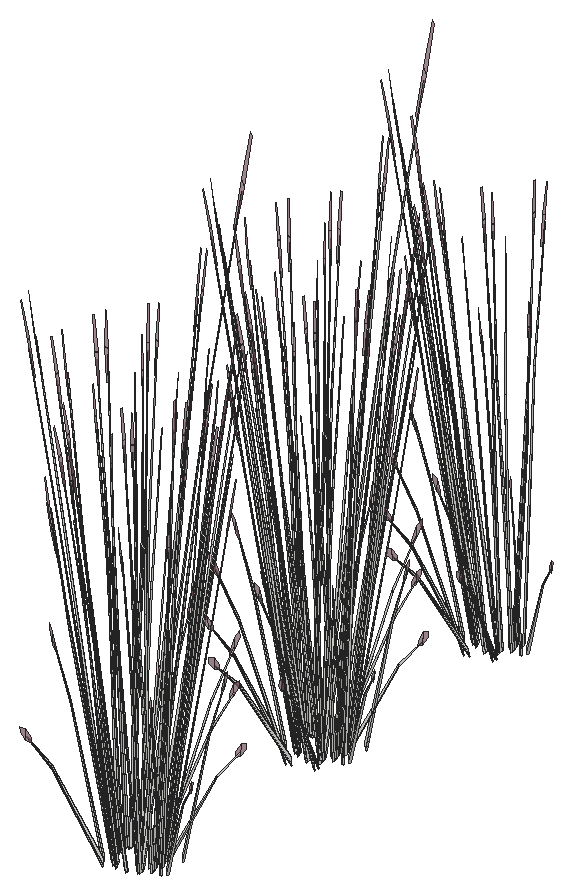
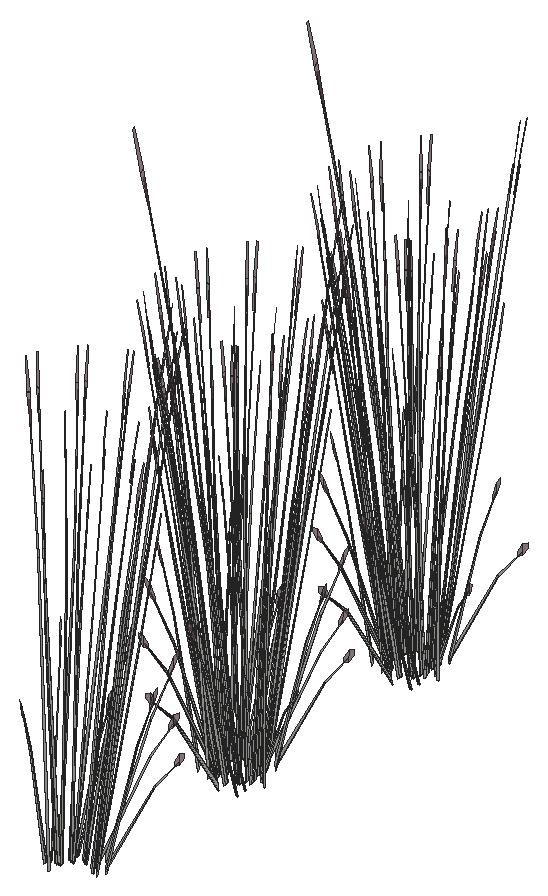
# SketchUp Ruby script. Lengths in inches.
U = 1.inch
M = Sketchup.active_model
def pt(a) = Geom::Point3d.new(a.map { |v| v * U })
def face(e, loops, mat)
  f = e.add_face(loops[0].map { |a| pt(a) })
  loops[1..].each { |l| e.add_face(l.map { |a| pt(a) }).erase! }
  f.material = f.back_material = mat if mat
  f
end
# faces: each face lists its corners as indices into pts; further lists are holes
def faces(e, pts, list, mat = nil) = list.each { |f| face(e, (f[0].is_a?(Array) ? f : [f]).map { |l| l.map { |i| pts[i] } }, mat) }
# xy, xz, yz: faces in a plane at the given z, y or x. An outline is a flat list of corners, or four numbers for a rectangle; further outlines are holes
def ring(l) = l.size == 4 ? [[l[0], l[1]], [l[2], l[1]], [l[2], l[3]], [l[0], l[3]]] : l.each_slice(2).to_a
def flat(e, list, mat, &to3) = list.each { |f| face(e, (f[0].is_a?(Array) ? f : [f]).map { |l| ring(l).map { |u, v| to3.(u, v) } }, mat) }
def xy(e, z, list, mat = nil) = flat(e, list, mat) { |x, y| [x, y, z] }
def xz(e, y, list, mat = nil) = flat(e, list, mat) { |x, z| [x, y, z] }
def yz(e, x, list, mat = nil) = flat(e, list, mat) { |y, z| [x, y, z] }
def lines(e, pts, list) = list.each { |a, b| e.add_line(pt(pts[a]), pt(pts[b])) }
# prism: a flat outline (further loops are holes) pulled along v
def prism(e, loops, v, mat = nil)
  f = face(e, loops, mat); d = Geom::Vector3d.new(v.map { |x| x * U })
  f.pushpull(f.normal.samedirection?(d) ? d.length : -d.length)
end
def box(e, o, s, mat = nil) = prism(e, [[o, [o[0] + s[0], o[1], o[2]], [o[0] + s[0], o[1] + s[1], o[2]], [o[0], o[1] + s[1], o[2]]]], [0, 0, s[2]], mat)
def at(x, y, z, deg = 0) = Geom::Transformation.translation(pt([x, y, z])) * Geom::Transformation.rotation(ORIGIN, Z_AXIS, deg.degrees)
def axes(o, x, y, z) = Geom::Transformation.new([*x, 0, *y, 0, *z, 0, *pt(o).to_a, 1])
def part(name) = M.definitions.add(name)
# library, detail: a bought-in or finely detailed component or shape, given as its bounding box
def library(name, o, s) = part(name).tap { |d| box(d.entities, o, s) }
def detail(e, o, s) = box(e.add_group.entities, o, s)
def put(e, d, t, mat = nil) = e.add_instance(d, t).tap { |i| i.material = mat if mat }
def group(e, t, mat = nil) = e.add_group.tap { |g| g.transformation = t; g.material = mat if mat }.entities
root = M.entities
M.materials.add("LightPink_Translucent").color = [144, 107, 117]
M.materials["LightPink_Translucent"].alpha = 0.75
c1 = part("blade")
p = [[2.15,0.21,22],[0,0.17,0],[0.09,0.45,0],[2.18,0.31,22],[2.29,0.31,22],[0.38,0.45,0],
  [2.48,0.24,33],[2.49,0.24,33],[2.48,0.22,33]]
faces(c1.entities,p,[[0,1,2,3],[4,5,2,3],[6,3,4,7],[8,0,3,6]])
c2 = part("seeds")
p = [[0.3,-0.1,1.38],[-0.01,-0.03,1.59],[-0.01,-0.03,0.03],[0.14,-0.07,-0.07],[0.29,-0.03,3],[0.15,0.01,3.11]]
faces(c2.entities,p,[[0,1,2,3],[1,0,4,5]],"LightPink_Translucent")
c3 = part("blade with seeds")
put(c3.entities,c1,at(0,0,0))
put(c3.entities,c2,axes([2.4,0.25,30.99],[1.5799,-0.05474,1.17369],[-0.12525,1.92788,0.29478],[-0.07173,-0.02425,1.56792]))
put(root,c3,axes([402.43,636.52,4.73],[0.26007,-0.1585,0.0643],[0.12729,0.28902,0.50621],[-0.02512,-0.1274,0.77189]))
put(root,c3,axes([401.54,636.56,4.73],[0.16041,-0.29625,0.0643],[0.22843,0.17248,0.50621],[-0.07385,-0.09498,0.77189]))
put(root,c3,axes([402.33,636.84,5.05],[-0.1064,0.35863,0.35414],[-0.31043,-0.1046,-0.4572],[-0.02846,-0.14439,0.87481]))
put(root,c3,axes([403.125,636.99,4.73],[0.25132,0.3182,0.48003],[-0.2669,0.27442,0.3958],[0.04636,-0.14929,0.9933]))
put(root,c3,axes([401.61,636.53,5.43],[-0.23555,0.44708,-0.13619],[-0.34112,-0.25757,-0.75594],[-0.11858,-0.12631,1.14864]))
put(root,c3,axes([403.22,637.02,4.73],[0.29004,0.02173,0.0643],[-0.00795,0.32812,0.50621],[0.03035,-0.12569,0.77189]))
put(root,c3,axes([403,637.24,5.05],[-0.23881,0.24554,0.35414],[-0.22606,-0.28036,-0.4572],[0.0344,-0.14245,0.87481]))
put(root,c3,axes([400.71,636.4,4.72],[-0.07594,-0.00329,1.74944],[-0.24177,0.32918,-0.27667],[-0.129,-0.06726,0.14031]))
put(root,c3,axes([403.58,638.04,5.03],[-0.32648,-0.25715,-0.1216],[0.18809,-0.3724,-0.67495],[0.09224,-0.12945,1.02557]))
put(root,c3,axes([401.59,636.9,5.05],[0.05451,0.37564,0.35414],[-0.31161,0.09919,-0.4572],[-0.0837,-0.10765,0.87481]))
put(root,c3,axes([400.65,637.15,5.09],[0.29147,-0.34417,0.53763],[0.25138,0.3655,0.4433],[-0.13675,-0.06349,1.11249]))
put(root,c3,axes([404.38,637.93,4.71],[-0.0461,-0.00354,1.77383],[-0.19143,-0.37951,-0.16761],[0.07688,-0.12478,0.31391]))
put(root,c3,axes([400.78,637.14,4.73],[0.01777,-0.35463,0.0643],[0.26836,0.00972,0.50621],[-0.1028,-0.03711,0.77189]))
put(root,c3,axes([403.42,638,5.05],[-0.30722,0.06665,0.35414],[-0.08112,-0.381,-0.4572],[0.08804,-0.10234,0.87481]))
put(root,c3,axes([403.7,637.94,4.73],[0.2423,0.19613,0.0643],[-0.14107,0.2793,0.50621],[0.07768,-0.0903,0.77189]))
put(root,c3,axes([403.63,637.86,4.73],[0.08753,0.42921,0.48003],[-0.34336,0.07449,0.3958],[0.1012,-0.10094,0.9933]))
put(root,c3,axes([404.55,638.38,4.72],[0.04898,-0.07104,1.74944],[-0.06269,-0.43574,-0.27667],[0.12289,-0.08262,0.14031]))
put(root,c3,axes([400.42,636.68,4.71],[0.02617,0.04654,1.77383],[-0.12614,0.41836,-0.16761],[-0.12775,0.00303,0.31391]))
put(root,c3,axes([400.97,637.41,5.05],[0.20082,0.29199,0.35414],[-0.2293,0.2764,-0.4572],[-0.1165,-0.04206,0.87481]))
put(root,c3,axes([400.91,637.22,5.03],[-0.0189,0.47427,-0.1216],[-0.35781,-0.01296,-0.67495],[-0.13781,-0.03295,1.02557]))
put(root,c3,axes([403.59,639.04,5.03],[-0.17758,-0.42229,-0.1216],[0.31518,-0.20752,-0.67495],[0.13282,-0.05572,1.02557]))
put(root,c3,axes([403.47,638.91,5.05],[-0.29332,-0.1301,0.35414],[0.08555,-0.37955,-0.4572],[0.11809,-0.0348,0.87481]))
put(root,c3,axes([400.4,638.22,4.73],[0.09971,-0.42522,0.48003],[0.32782,0.1454,0.3958],[-0.12892,0.02555,0.9933]))
put(root,c3,axes([400.37,638.11,4.73],[-0.12963,-0.31798,0.0643],[0.23638,-0.15564,0.50621],[-0.1042,0.03071,0.77189]))
put(root,c3,axes([403.73,639.03,4.73],[0.12963,0.31798,0.0643],[-0.23638,0.15564,0.50621],[0.1042,-0.03071,0.77189]))
put(root,c3,axes([403.71,638.92,4.73],[-0.09971,0.42522,0.48003],[-0.32782,-0.1454,0.3958],[0.12892,-0.02555,0.9933]))
put(root,c3,axes([400.64,638.23,5.05],[0.29332,0.1301,0.35414],[-0.08555,0.37955,-0.4572],[-0.11809,0.0348,0.87481]))
put(root,c3,axes([404.3,640.3,4.71],[-0.03191,-0.04083,1.77383],[0.06981,-0.43764,-0.16761],[0.12571,-0.02796,0.31391]))
put(root,c3,axes([400.14,638.52,4.72],[-0.05763,0.06055,1.74944],[0.0049,0.44239,-0.27667],[-0.13211,0.05753,0.14031]))
put(root,c3,axes([400.51,638.1,5.03],[0.17758,0.42229,-0.1216],[-0.31518,0.20752,-0.67495],[-0.13282,0.05572,1.02557]))
put(root,c3,axes([403.19,639.92,5.03],[0.0189,-0.47427,-0.1216],[0.35781,0.01296,-0.67495],[0.13781,0.03295,1.02557]))
put(root,c3,axes([403.14,639.73,5.05],[-0.20082,-0.29199,0.35414],[0.2293,-0.2764,-0.4572],[0.1165,0.04206,0.87481]))
put(root,c3,axes([403.5,639.63,4.72],[0.07571,-0.00789,1.74944],[0.20767,-0.36231,-0.27667],[0.13467,0.04783,0.14031]))
put(root,c3,axes([400.47,639.28,4.73],[-0.08753,-0.42921,0.48003],[0.34336,-0.07449,0.3958],[-0.1012,0.10094,0.9933]))
put(root,c3,axes([400.41,639.2,4.73],[-0.2423,-0.19613,0.0643],[0.14107,-0.2793,0.50621],[-0.07768,0.0903,0.77189]))
put(root,c3,axes([400.6875,639.14,5.05],[0.30722,-0.06665,0.35414],[0.08112,0.381,-0.4572],[-0.08804,0.10234,0.87481]))
put(root,c3,axes([399.5,638.97,4.71],[0.04504,0.01251,1.77383],[0.13934,0.41205,-0.16761],[-0.0922,0.10815,0.31391]))
put(root,c3,axes([403.32,640,4.73],[-0.01777,0.35463,0.0643],[-0.26836,-0.00972,0.50621],[0.1028,0.03711,0.77189]))
put(root,c3,axes([403.34,639.89,4.73],[-0.26024,0.30729,0.48003],[-0.22444,-0.32634,0.3958],[0.1221,0.05668,0.9933]))
put(root,c3,axes([399.99,640.22,5.65],[0.31145,0.12449,-0.06488],[-0.0958,0.38314,-0.29416],[-0.05094,0.05817,0.97024]))
put(root,c3,axes([402.52,640.24,5.05],[-0.05451,-0.37564,0.35414],[0.31161,-0.09919,-0.4572],[0.0837,0.10765,0.87481]))
put(root,c3,axes([402.72,638.08,4.47],[-0.30498,-0.24231,1.38283],[0.32203,-0.37727,0.59665],[0.0984,0.22736,1.33663]))
put(root,c3,axes([400.53,639.1,5.03],[0.32648,0.25715,-0.1216],[-0.18809,0.3724,-0.67495],[-0.09224,0.12945,1.02557]))
put(root,c3,axes([402.49,640.44,5.03],[0.21031,-0.39918,-0.1216],[0.30457,0.22997,-0.67495],[0.10587,0.11278,1.02557]))
put(root,c3,axes([401.1,639.9,5.05],[0.23881,-0.24554,0.35414],[0.22606,0.28036,-0.4572],[-0.0344,0.14245,0.87481]))
put(root,c3,axes([402.21,640.77,4.71],[0.00104,-0.05646,1.77383],[0.30246,-0.2491,-0.16761],[0.10506,0.08891,0.31391]))
put(root,c3,axes([400.88,640.12,4.73],[-0.29004,-0.02173,0.0643],[0.00795,-0.32812,0.50621],[-0.03035,0.12569,0.77189]))
put(root,c3,axes([400.98,640.15,4.73],[-0.25132,-0.3182,0.48003],[0.2669,-0.27442,0.3958],[-0.04636,0.14929,0.9933]))
put(root,c3,axes([401.77,640.3,5.05],[0.1064,-0.35863,0.35414],[0.31043,0.1046,-0.4572],[0.02846,0.14439,0.87481]))
put(root,c3,axes([402.56,640.58,4.73],[-0.16041,0.29625,0.0643],[-0.22843,-0.17248,0.50621],[0.07385,0.09498,0.77189]))
put(root,c3,axes([402.1875,641.58,5.65],[0.2439,-0.26754,-0.06488],[0.22348,0.29302,-0.29416],[0.01573,0.08303,0.97024]))
put(root,c3,axes([402.63,640.5,4.73],[-0.35104,0.10702,0.48003],[-0.06092,-0.41983,0.3958],[0.08256,0.12373,0.9933]))
put(root,c3,axes([401.67,640.625,4.73],[-0.26007,0.1585,0.0643],[-0.12729,-0.28902,0.50621],[0.02512,0.1274,0.77189]))
put(root,c3,axes([400.15,640.17,4.72],[-0.00877,0.09229,1.74944],[0.24897,0.32105,-0.27667],[-0.06518,0.15182,0.14031]))
put(root,c3,axes([400.95,639.96,5.4],[0.3879,0.02311,-0.13498],[-0.0106,0.43749,-0.74919],[-0.02694,0.1685,1.13838]))
put(root,c3,axes([401.67,640.45,5.03],[0.34538,-0.21713,-0.1216],[0.16972,0.38536,-0.67495],[0.04557,0.16239,1.02557]))
put(root,c3,axes([401.77,640.6,5.0625],[-0.34777,-0.12192,0.53283],[0.11892,-0.40083,0.43934],[0.0209,0.15763,1.10256]))
put(root,c3,axes([400.125,641.12,4.71],[0.04004,-0.02816,1.77383],[0.33095,0.18728,-0.16761],[-0.00778,0.15594,0.31391]))
put(root,c3,axes([401.58,641.3125,4.72],[0.04474,0.0751,1.74944],[0.36104,0.0295,-0.27667],[0.03631,0.16562,0.14031]))
put(root,c3,axes([401.89,654.35,4.72],[-0.05398,-0.06539,1.74944],[-0.36026,0.04145,-0.27667],[-0.0575,-0.15639,0.14031]))
put(root,c3,axes([403.51,655.16,4.72],[-0.00341,-0.09282,1.74944],[-0.28775,-0.26825,-0.27667],[0.04449,-0.16261,0.14031]))
put(root,c3,axes([403.43,654.82,4.71],[-0.03584,0.03562,1.77383],[-0.35118,-0.12018,-0.16761],[-0.01271,-0.15545,0.31391]))
put(root,c3,axes([401.52,654.14,4.71],[-0.00658,0.0559,1.77383],[-0.32474,0.20287,-0.16761],[-0.09556,-0.1037,0.31391]))
put(root,c3,axes([401.45,655.13,5.09],[0.39316,-0.11987,0.53763],[0.06823,0.47021,0.4433],[-0.09247,-0.13858,1.11249]))
put(root,c3,axes([402.34,655.22,4.73],[0.34777,0.12192,0.48003],[-0.11892,0.40083,0.3958],[-0.0209,-0.15763,0.9933]))
put(root,c3,axes([402.4375,655.36,5.03],[-0.34538,0.21713,-0.1216],[-0.16972,-0.38536,-0.67495],[-0.04557,-0.16239,1.02557]))
put(root,c3,axes([403.15,655.85,5.03],[-0.3879,-0.02311,-0.1216],[0.0106,-0.43749,-0.67495],[0.02694,-0.1685,1.02557]))
put(root,c3,axes([402.43,655.19,4.73],[0.26007,-0.1585,0.0643],[0.12729,0.28902,0.50621],[-0.02512,-0.1274,0.77189]))
put(root,c3,axes([401.54,655.23,4.73],[0.16041,-0.29625,0.0643],[0.22843,0.17248,0.50621],[-0.07385,-0.09498,0.77189]))
put(root,c3,axes([402.33,655.51,5.05],[-0.1064,0.35863,0.35414],[-0.31043,-0.1046,-0.4572],[-0.02846,-0.14439,0.87481]))
put(root,c3,axes([403.125,655.67,4.73],[0.25132,0.3182,0.48003],[-0.2669,0.27442,0.3958],[0.04636,-0.14929,0.9933]))
put(root,c3,axes([401.61,655.2,5.43],[-0.23555,0.44708,-0.13619],[-0.34112,-0.25757,-0.75594],[-0.11858,-0.12631,1.14864]))
put(root,c3,axes([403.22,655.7,4.73],[0.29004,0.02173,0.0643],[-0.00795,0.32812,0.50621],[0.03035,-0.12569,0.77189]))
put(root,c3,axes([403,655.92,5.05],[-0.23881,0.24554,0.35414],[-0.22606,-0.28036,-0.4572],[0.0344,-0.14245,0.87481]))
put(root,c3,axes([400.71,655.07,4.72],[-0.07594,-0.00329,1.74944],[-0.24177,0.32918,-0.27667],[-0.129,-0.06726,0.14031]))
put(root,c3,axes([403.58,656.71,5.03],[-0.32648,-0.25715,-0.1216],[0.18809,-0.3724,-0.67495],[0.09224,-0.12945,1.02557]))
put(root,c3,axes([401.59,655.57,5.05],[0.05451,0.37564,0.35414],[-0.31161,0.09919,-0.4572],[-0.0837,-0.10765,0.87481]))
put(root,c3,axes([400.65,655.82,5.09],[0.29147,-0.34417,0.53763],[0.25138,0.3655,0.4433],[-0.13675,-0.06349,1.11249]))
put(root,c3,axes([404.38,656.6,4.71],[-0.0461,-0.00354,1.77383],[-0.19143,-0.37951,-0.16761],[0.07688,-0.12478,0.31391]))
put(root,c3,axes([400.78,655.82,4.73],[0.01777,-0.35463,0.0643],[0.26836,0.00972,0.50621],[-0.1028,-0.03711,0.77189]))
put(root,c3,axes([403.42,656.68,5.05],[-0.30722,0.06665,0.35414],[-0.08112,-0.381,-0.4572],[0.08804,-0.10234,0.87481]))
put(root,c3,axes([403.7,656.62,4.73],[0.2423,0.19613,0.0643],[-0.14107,0.2793,0.50621],[0.07768,-0.0903,0.77189]))
put(root,c3,axes([403.63,656.53,4.73],[0.08753,0.42921,0.48003],[-0.34336,0.07449,0.3958],[0.1012,-0.10094,0.9933]))
put(root,c3,axes([404.55,657.05,4.72],[0.04898,-0.07104,1.74944],[-0.06269,-0.43574,-0.27667],[0.12289,-0.08262,0.14031]))
put(root,c3,axes([400.42,655.35,4.71],[0.02617,0.04654,1.77383],[-0.12614,0.41836,-0.16761],[-0.12775,0.00303,0.31391]))
put(root,c3,axes([400.97,656.08,5.05],[0.20082,0.29199,0.35414],[-0.2293,0.2764,-0.4572],[-0.1165,-0.04206,0.87481]))
put(root,c3,axes([400.91,655.9,5.03],[-0.0189,0.47427,-0.1216],[-0.35781,-0.01296,-0.67495],[-0.13781,-0.03295,1.02557]))
put(root,c3,axes([403.59,657.72,5.03],[-0.17758,-0.42229,-0.1216],[0.31518,-0.20752,-0.67495],[0.13282,-0.05572,1.02557]))
put(root,c3,axes([403.47,657.59,5.05],[-0.29332,-0.1301,0.35414],[0.08555,-0.37955,-0.4572],[0.11809,-0.0348,0.87481]))
put(root,c3,axes([400.4,656.9,4.73],[0.09971,-0.42522,0.48003],[0.32782,0.1454,0.3958],[-0.12892,0.02555,0.9933]))
put(root,c3,axes([400.37,656.78,4.73],[-0.12963,-0.31798,0.0643],[0.23638,-0.15564,0.50621],[-0.1042,0.03071,0.77189]))
put(root,c3,axes([403.73,657.71,4.73],[0.12963,0.31798,0.0643],[-0.23638,0.15564,0.50621],[0.1042,-0.03071,0.77189]))
put(root,c3,axes([403.71,657.59,4.73],[-0.09971,0.42522,0.48003],[-0.32782,-0.1454,0.3958],[0.12892,-0.02555,0.9933]))
put(root,c3,axes([400.64,656.9,5.05],[0.29332,0.1301,0.35414],[-0.08555,0.37955,-0.4572],[-0.11809,0.0348,0.87481]))
put(root,c3,axes([404.3,658.97,4.71],[-0.03191,-0.04083,1.77383],[0.06981,-0.43764,-0.16761],[0.12571,-0.02796,0.31391]))
put(root,c3,axes([400.14,657.19,4.72],[-0.05763,0.06055,1.74944],[0.0049,0.44239,-0.27667],[-0.13211,0.05753,0.14031]))
put(root,c3,axes([400.51,656.77,5.03],[0.17758,0.42229,-0.1216],[-0.31518,0.20752,-0.67495],[-0.13282,0.05572,1.02557]))
put(root,c3,axes([403.19,658.59,5.03],[0.0189,-0.47427,-0.1216],[0.35781,0.01296,-0.67495],[0.13781,0.03295,1.02557]))
put(root,c3,axes([403.14,658.41,5.05],[-0.20082,-0.29199,0.35414],[0.2293,-0.2764,-0.4572],[0.1165,0.04206,0.87481]))
put(root,c3,axes([403.5,658.31,4.72],[0.07571,-0.00789,1.74944],[0.20767,-0.36231,-0.27667],[0.13467,0.04783,0.14031]))
put(root,c3,axes([400.47,657.95,4.73],[-0.08753,-0.42921,0.48003],[0.34336,-0.07449,0.3958],[-0.1012,0.10094,0.9933]))
put(root,c3,axes([400.41,657.87,4.73],[-0.2423,-0.19613,0.0643],[0.14107,-0.2793,0.50621],[-0.07768,0.0903,0.77189]))
put(root,c3,axes([400.6875,657.8125,5.05],[0.30722,-0.06665,0.35414],[0.08112,0.381,-0.4572],[-0.08804,0.10234,0.87481]))
put(root,c3,axes([399.5,657.64,4.71],[0.04504,0.01251,1.77383],[0.13934,0.41205,-0.16761],[-0.0922,0.10815,0.31391]))
put(root,c3,axes([403.32,658.67,4.73],[-0.01777,0.35463,0.0643],[-0.26836,-0.00972,0.50621],[0.1028,0.03711,0.77189]))
put(root,c3,axes([403.34,658.56,4.73],[-0.26024,0.30729,0.48003],[-0.22444,-0.32634,0.3958],[0.1221,0.05668,0.9933]))
put(root,c3,axes([399.99,658.89,5.65],[0.31145,0.12449,-0.06488],[-0.0958,0.38314,-0.29416],[-0.05094,0.05817,0.97024]))
put(root,c3,axes([402.52,658.91,5.05],[-0.05451,-0.37564,0.35414],[0.31161,-0.09919,-0.4572],[0.0837,0.10765,0.87481]))
put(root,c3,axes([402.72,656.75,4.47],[-0.30498,-0.24231,1.38283],[0.32203,-0.37727,0.59665],[0.0984,0.22736,1.33663]))
put(root,c3,axes([400.53,657.78,5.03],[0.32648,0.25715,-0.1216],[-0.18809,0.3724,-0.67495],[-0.09224,0.12945,1.02557]))
put(root,c3,axes([402.49,659.11,5.03],[0.21031,-0.39918,-0.1216],[0.30457,0.22997,-0.67495],[0.10587,0.11278,1.02557]))
put(root,c3,axes([401.1,658.57,5.05],[0.23881,-0.24554,0.35414],[0.22606,0.28036,-0.4572],[-0.0344,0.14245,0.87481]))
put(root,c3,axes([402.21,659.44,4.71],[0.00104,-0.05646,1.77383],[0.30246,-0.2491,-0.16761],[0.10506,0.08891,0.31391]))
put(root,c3,axes([400.88,658.79,4.73],[-0.29004,-0.02173,0.0643],[0.00795,-0.32812,0.50621],[-0.03035,0.12569,0.77189]))
put(root,c3,axes([400.98,658.82,4.73],[-0.25132,-0.3182,0.48003],[0.2669,-0.27442,0.3958],[-0.04636,0.14929,0.9933]))
put(root,c3,axes([401.77,658.97,5.05],[0.1064,-0.35863,0.35414],[0.31043,0.1046,-0.4572],[0.02846,0.14439,0.87481]))
put(root,c3,axes([402.56,659.26,4.73],[-0.16041,0.29625,0.0643],[-0.22843,-0.17248,0.50621],[0.07385,0.09498,0.77189]))
put(root,c3,axes([402.1875,660.25,5.65],[0.2439,-0.26754,-0.06488],[0.22348,0.29302,-0.29416],[0.01573,0.08303,0.97024]))
put(root,c3,axes([402.63,659.17,4.73],[-0.35104,0.10702,0.48003],[-0.06092,-0.41983,0.3958],[0.08256,0.12373,0.9933]))
put(root,c3,axes([401.67,659.3,4.73],[-0.26007,0.1585,0.0643],[-0.12729,-0.28902,0.50621],[0.02512,0.1274,0.77189]))
put(root,c3,axes([400.15,658.85,4.72],[-0.00877,0.09229,1.74944],[0.24897,0.32105,-0.27667],[-0.06518,0.15182,0.14031]))
put(root,c3,axes([400.95,658.64,5.4],[0.3879,0.02311,-0.13498],[-0.0106,0.43749,-0.74919],[-0.02694,0.1685,1.13838]))
put(root,c3,axes([401.67,659.125,5.03],[0.34538,-0.21713,-0.1216],[0.16972,0.38536,-0.67495],[0.04557,0.16239,1.02557]))
put(root,c3,axes([401.77,659.27,5.0625],[-0.34777,-0.12192,0.53283],[0.11892,-0.40083,0.43934],[0.0209,0.15763,1.10256]))
put(root,c3,axes([400.125,659.79,4.71],[0.04004,-0.02816,1.77383],[0.33095,0.18728,-0.16761],[-0.00778,0.15594,0.31391]))
put(root,c3,axes([401.58,659.99,4.72],[0.04474,0.0751,1.74944],[0.36104,0.0295,-0.27667],[0.03631,0.16562,0.14031]))
put(root,c3,axes([401.89,672.57,4.72],[-0.05398,-0.06539,1.74944],[-0.36026,0.04145,-0.27667],[-0.0575,-0.15639,0.14031]))
put(root,c3,axes([403.51,673.37,4.72],[-0.00341,-0.09282,1.74944],[-0.28775,-0.26825,-0.27667],[0.04449,-0.16261,0.14031]))
put(root,c3,axes([403.43,673.04,4.71],[-0.03584,0.03562,1.77383],[-0.35118,-0.12018,-0.16761],[-0.01271,-0.15545,0.31391]))
put(root,c3,axes([401.52,672.36,4.71],[-0.00658,0.0559,1.77383],[-0.32474,0.20287,-0.16761],[-0.09556,-0.1037,0.31391]))
put(root,c3,axes([401.45,673.35,5.09],[0.39316,-0.11987,0.53763],[0.06823,0.47021,0.4433],[-0.09247,-0.13858,1.11249]))
put(root,c3,axes([402.34,673.44,4.73],[0.34777,0.12192,0.48003],[-0.11892,0.40083,0.3958],[-0.0209,-0.15763,0.9933]))
put(root,c3,axes([402.4375,673.58,5.03],[-0.34538,0.21713,-0.1216],[-0.16972,-0.38536,-0.67495],[-0.04557,-0.16239,1.02557]))
put(root,c3,axes([403.15,674.07,5.03],[-0.3879,-0.02311,-0.1216],[0.0106,-0.43749,-0.67495],[0.02694,-0.1685,1.02557]))
put(root,c3,axes([402.43,673.4,4.73],[0.26007,-0.1585,0.0643],[0.12729,0.28902,0.50621],[-0.02512,-0.1274,0.77189]))
put(root,c3,axes([401.54,673.45,4.73],[0.16041,-0.29625,0.0643],[0.22843,0.17248,0.50621],[-0.07385,-0.09498,0.77189]))
put(root,c3,axes([402.33,673.73,5.05],[-0.1064,0.35863,0.35414],[-0.31043,-0.1046,-0.4572],[-0.02846,-0.14439,0.87481]))
put(root,c3,axes([403.125,673.88,4.73],[0.25132,0.3182,0.48003],[-0.2669,0.27442,0.3958],[0.04636,-0.14929,0.9933]))
put(root,c3,axes([401.61,673.42,5.43],[-0.23555,0.44708,-0.13619],[-0.34112,-0.25757,-0.75594],[-0.11858,-0.12631,1.14864]))
put(root,c3,axes([403.22,673.91,4.73],[0.29004,0.02173,0.0643],[-0.00795,0.32812,0.50621],[0.03035,-0.12569,0.77189]))
put(root,c3,axes([403,674.13,5.05],[-0.23881,0.24554,0.35414],[-0.22606,-0.28036,-0.4572],[0.0344,-0.14245,0.87481]))
put(root,c3,axes([400.71,673.29,4.72],[-0.07594,-0.00329,1.74944],[-0.24177,0.32918,-0.27667],[-0.129,-0.06726,0.14031]))
put(root,c3,axes([403.58,674.93,5.03],[-0.32648,-0.25715,-0.1216],[0.18809,-0.3724,-0.67495],[0.09224,-0.12945,1.02557]))
put(root,c3,axes([401.59,673.79,5.05],[0.05451,0.37564,0.35414],[-0.31161,0.09919,-0.4572],[-0.0837,-0.10765,0.87481]))
put(root,c3,axes([400.65,674.03,5.09],[0.29147,-0.34417,0.53763],[0.25138,0.3655,0.4433],[-0.13675,-0.06349,1.11249]))
put(root,c3,axes([404.38,674.82,4.71],[-0.0461,-0.00354,1.77383],[-0.19143,-0.37951,-0.16761],[0.07688,-0.12478,0.31391]))
put(root,c3,axes([400.78,674.03,4.73],[0.01777,-0.35463,0.0643],[0.26836,0.00972,0.50621],[-0.1028,-0.03711,0.77189]))
put(root,c3,axes([403.42,674.89,5.05],[-0.30722,0.06665,0.35414],[-0.08112,-0.381,-0.4572],[0.08804,-0.10234,0.87481]))
put(root,c3,axes([403.7,674.83,4.73],[0.2423,0.19613,0.0643],[-0.14107,0.2793,0.50621],[0.07768,-0.0903,0.77189]))
put(root,c3,axes([403.63,674.75,4.73],[0.08753,0.42921,0.48003],[-0.34336,0.07449,0.3958],[0.1012,-0.10094,0.9933]))
put(root,c3,axes([404.55,675.27,4.72],[0.04898,-0.07104,1.74944],[-0.06269,-0.43574,-0.27667],[0.12289,-0.08262,0.14031]))
put(root,c3,axes([400.42,673.57,4.71],[0.02617,0.04654,1.77383],[-0.12614,0.41836,-0.16761],[-0.12775,0.00303,0.31391]))
put(root,c3,axes([400.97,674.3,5.05],[0.20082,0.29199,0.35414],[-0.2293,0.2764,-0.4572],[-0.1165,-0.04206,0.87481]))
put(root,c3,axes([400.91,674.11,5.03],[-0.0189,0.47427,-0.1216],[-0.35781,-0.01296,-0.67495],[-0.13781,-0.03295,1.02557]))
put(root,c3,axes([403.59,675.93,5.03],[-0.17758,-0.42229,-0.1216],[0.31518,-0.20752,-0.67495],[0.13282,-0.05572,1.02557]))
